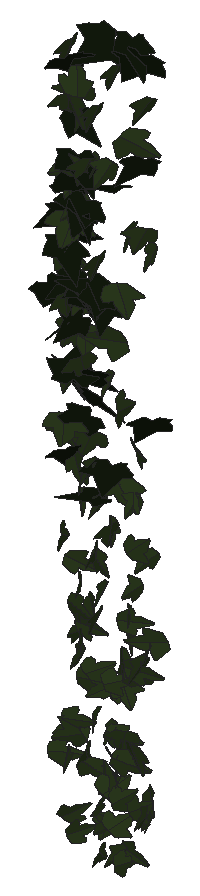
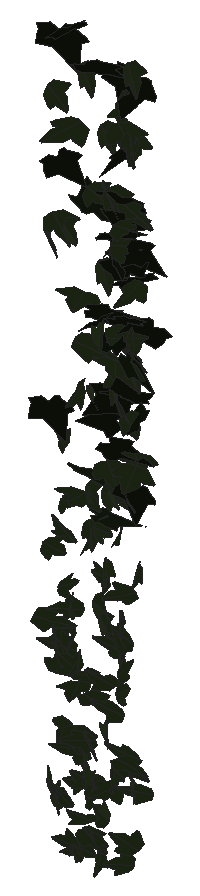
# SketchUp Ruby script. Lengths in inches.
U = 1.inch
M = Sketchup.active_model
def pt(a) = Geom::Point3d.new(a.map { |v| v * U })
def face(e, loops, mat)
  f = e.add_face(loops[0].map { |a| pt(a) })
  loops[1..].each { |l| e.add_face(l.map { |a| pt(a) }).erase! }
  f.material = f.back_material = mat if mat
  f
end
# faces: each face lists its corners as indices into pts; further lists are holes
def faces(e, pts, list, mat = nil) = list.each { |f| face(e, (f[0].is_a?(Array) ? f : [f]).map { |l| l.map { |i| pts[i] } }, mat) }
# xy, xz, yz: faces in a plane at the given z, y or x. An outline is a flat list of corners, or four numbers for a rectangle; further outlines are holes
def ring(l) = l.size == 4 ? [[l[0], l[1]], [l[2], l[1]], [l[2], l[3]], [l[0], l[3]]] : l.each_slice(2).to_a
def flat(e, list, mat, &to3) = list.each { |f| face(e, (f[0].is_a?(Array) ? f : [f]).map { |l| ring(l).map { |u, v| to3.(u, v) } }, mat) }
def xy(e, z, list, mat = nil) = flat(e, list, mat) { |x, y| [x, y, z] }
def xz(e, y, list, mat = nil) = flat(e, list, mat) { |x, z| [x, y, z] }
def yz(e, x, list, mat = nil) = flat(e, list, mat) { |y, z| [x, y, z] }
def lines(e, pts, list) = list.each { |a, b| e.add_line(pt(pts[a]), pt(pts[b])) }
# prism: a flat outline (further loops are holes) pulled along v
def prism(e, loops, v, mat = nil)
  f = face(e, loops, mat); d = Geom::Vector3d.new(v.map { |x| x * U })
  f.pushpull(f.normal.samedirection?(d) ? d.length : -d.length)
end
def box(e, o, s, mat = nil) = prism(e, [[o, [o[0] + s[0], o[1], o[2]], [o[0] + s[0], o[1] + s[1], o[2]], [o[0], o[1] + s[1], o[2]]]], [0, 0, s[2]], mat)
def at(x, y, z, deg = 0) = Geom::Transformation.translation(pt([x, y, z])) * Geom::Transformation.rotation(ORIGIN, Z_AXIS, deg.degrees)
def axes(o, x, y, z) = Geom::Transformation.new([*x, 0, *y, 0, *z, 0, *pt(o).to_a, 1])
def part(name) = M.definitions.add(name)
# library, detail: a bought-in or finely detailed component or shape, given as its bounding box
def library(name, o, s) = part(name).tap { |d| box(d.entities, o, s) }
def detail(e, o, s) = box(e.add_group.entities, o, s)
def put(e, d, t, mat = nil) = e.add_instance(d, t).tap { |i| i.material = mat if mat }
def group(e, t, mat = nil) = e.add_group.tap { |g| g.transformation = t; g.material = mat if mat }.entities
root = M.entities
M.materials.add("1026 AP 7946 SUNNY SIDE UP").color = [254, 231, 186]
M.materials.add("efeu1").color = [18, 25, 13]
M.materials.add("efeu2").color = [43, 57, 29]
c1 = part("ivyleaf_10")
p = [[0,0.5,-0.03],[-0.0625,2.02,-0.43],[-0.19,2.01,-0.46],[-0.54,1.05,-0.29],[-0.52,0.625,-0.18],[-0.83,0.76,-0.28],
  [-1.16,0.64,-0.33],[-1.15,0.33,-0.24],[-0.77,-0.39,0.02],[-0.3,-0.51,0.16],[0.04,-0.48,0.23],[-0.02,2.01,-0.4375],
  [-0.06,2.01,-0.43],[0.04,-0.49,0.23],[0.67,-0.49,0.14],[1.38,0.36,-0.2],[1.375,0.51,-0.24],[0.81,0.65,-0.19],
  [0.62,0.59,-0.15],[0.6,1.09,-0.28],[0.5,1.23,-0.31]]
faces(c1.entities,p,[[0,1,2,3,4,5,6,7,8,9,10],[11,12,0,13,14,15,16,17,18,19,20]],"efeu2")
c2 = part("ivyleaf_9")
p = [[1.54,2.16,1.25],[1.36,2.04,1.19],[-0.21,0.99,0.68],[-0.71,1.11,0.82],[-0.85,0.86,0.67],[-0.8,0.17,0.21],
  [-0.9,-0.01,0.1],[-0.67,-0.16,-0.02],[-0.08,-0.08,-0.05],[-0.03,-0.6,-0.4],[0.65,-0.88,-0.66],[0.83,-0.6,-0.49],
  [1.29,-0.42,-0.43],[1.8125,-0.07,-0.26],[1.21,0.44,0.15]]
faces(c2.entities,p,[[0,1,2,3,4,5,6,7,8,9,10,11,12,13,14]],"efeu1")
put(root,c1,axes([100.47,212.17,263.79],[-0.24039,0.02209,0.20935],[-0.32195,-0.07836,-0.13886],[0.08731,-0.22813,0.06438]),"1026 AP 7946 SUNNY SIDE UP")
put(root,c2,axes([99.98,211.93,261.11],[0.0239,-0.04755,-0.26687],[0.13435,0.23738,-0.04049],[0.40821,-0.07534,0.02895]),"1026 AP 7946 SUNNY SIDE UP")
put(root,c2,axes([100.4,212.09,262.84],[0.00155,0.07561,-0.24059],[-0.11917,-0.21559,-0.08063],[-0.38611,0.06685,0.02392]),"1026 AP 7946 SUNNY SIDE UP")
put(root,c2,axes([100.26,212.05,257.41],[0.11959,0.20678,-0.02726],[-0.00549,-0.02863,-0.23417],[-0.35421,0.07026,-0.00557]),"1026 AP 7946 SUNNY SIDE UP")
put(root,c2,axes([100.36,212.17,260.38],[-0.19771,0.17255,-0.11554],[0.07257,-0.10346,-0.2233],[-0.33987,-0.12247,0.01953]),"1026 AP 7946 SUNNY SIDE UP")
put(root,c1,axes([100.25,212.3,259.09],[-0.07215,-0.19809,0.09557],[0.0269,-0.09613,-0.21543],[0.36968,-0.03167,0.03433]),"1026 AP 7946 SUNNY SIDE UP")
put(root,c1,axes([100.21,212.19,257.9],[-0.32784,-0.10769,-0.06],[0.09966,0.00208,-0.24019],[0.16417,-0.2163,0.02598]),"1026 AP 7946 SUNNY SIDE UP")
put(root,c1,axes([100.26,211.95,255.57],[0.04261,-0.11798,-0.19372],[0.01525,0.18922,-0.12019],[0.34784,0.00616,0.029]),"1026 AP 7946 SUNNY SIDE UP")
put(root,c1,axes([100.26,212.12,265.35],[-0.149,-0.21531,-0.06932],[0.04877,0.05516,-0.24808],[0.37718,-0.09219,0.00469]),"1026 AP 7946 SUNNY SIDE UP")
put(root,c2,axes([100.03,212.26,259.12],[0.16229,-0.17368,0.11092],[0.07726,-0.09575,-0.2135],[0.33654,0.10573,-0.00448]),"1026 AP 7946 SUNNY SIDE UP")
put(root,c1,axes([100.07,212,250.61],[0.04726,-0.03496,-0.20865],[0.31184,0.05795,0.02037],[0.08369,-0.19618,0.04191]),"1026 AP 7946 SUNNY SIDE UP")
put(root,c1,axes([100.29,212,260.91],[-0.0584,-0.23989,-0.06459],[0.08038,0.05026,-0.25542],[0.41085,-0.04393,0.04079]),"1026 AP 7946 SUNNY SIDE UP")
put(root,c1,axes([100.34,212.1,260.19],[0.29929,-0.15384,-0.0563],[-0.03832,0.0507,-0.2486],[0.27222,0.17628,0.0269]),"1026 AP 7946 SUNNY SIDE UP")
put(root,c1,axes([100.56,212.04,251.13],[-0.15865,-0.02106,0.18555],[-0.25796,-0.07753,-0.1044],[0.12193,-0.19145,0.02055]),"1026 AP 7946 SUNNY SIDE UP")
put(root,c1,axes([100.27,212,258.12],[0.35327,0.11008,-0.0093],[0.00151,-0.02324,-0.25137],[-0.18764,0.20705,-0.01953]),"1026 AP 7946 SUNNY SIDE UP")
put(root,c1,axes([100.47,212.24,265.53],[-0.2725,-0.1754,0.07998],[-0.07203,-0.0654,-0.25513],[0.3171,-0.16559,0.01078]),"1026 AP 7946 SUNNY SIDE UP")
put(root,c1,axes([100.48,212.18,251.27],[0.22898,0.02611,-0.15658],[-0.22621,-0.05286,-0.15151],[-0.08799,0.20386,-0.01794]),"1026 AP 7946 SUNNY SIDE UP")
put(root,c1,axes([100.4,212.39,263.43],[-0.14982,-0.09397,0.20911],[0.02605,-0.22348,-0.09962],[0.3515,-0.02349,0.09651]),"1026 AP 7946 SUNNY SIDE UP")
put(root,c1,axes([100.46,211.84,250.5],[0.13131,-0.0727,0.19088],[-0.16696,0.15421,0.11228],[-0.26543,-0.13296,0.0238]),"1026 AP 7946 SUNNY SIDE UP")
put(root,c1,axes([100.65,212.21,260.78],[-0.07244,-0.03101,-0.23099],[-0.35299,-0.05878,0.05235],[-0.10871,0.21153,-0.01608]),"1026 AP 7946 SUNNY SIDE UP")
put(root,c2,axes([100.5625,212.23,261.22],[-0.33259,-0.07967,0.07775],[-0.09386,-0.0575,-0.22484],[0.15848,-0.20126,0.02999]),"1026 AP 7946 SUNNY SIDE UP")
put(root,c1,axes([100.58,212.04,265.14],[0.11068,-0.10389,-0.24427],[-0.18526,0.19894,-0.12835],[0.38082,0.12697,0.00855]),"1026 AP 7946 SUNNY SIDE UP")
put(root,c1,axes([100.32,211.96,261.91],[-0.07184,-0.17471,-0.19224],[0.19427,0.14977,-0.17567],[0.35059,-0.11879,0.05795]),"1026 AP 7946 SUNNY SIDE UP")
put(root,c1,axes([100.48,211.93,266.74],[-0.01419,-0.25609,-0.00995],[0.00654,0.00583,-0.2742],[0.43479,-0.00845,0.0038]),"1026 AP 7946 SUNNY SIDE UP")
put(root,c2,axes([100.29,212.04,263.29],[-0.0241,-0.02577,0.25431],[0.35854,0.11061,0.02787],[-0.19084,0.21107,0.02024]),"1026 AP 7946 SUNNY SIDE UP")
put(root,c1,axes([100.49,212.33,262.94],[-0.0328,-0.08521,0.26333],[0.01701,-0.25692,-0.08866],[0.42405,0.00371,0.02392]),"1026 AP 7946 SUNNY SIDE UP")
put(root,c1,axes([100.42,212.29,253.32],[-0.01623,0.05009,0.20745],[0.0955,-0.19176,0.0513],[0.31153,0.06139,-0.00492]),"1026 AP 7946 SUNNY SIDE UP")
put(root,c1,axes([100.43,212.01,262.68],[0.40722,0.09065,-0.04278],[-0.05012,-0.03574,-0.28189],[-0.14891,0.25992,-0.02211]),"1026 AP 7946 SUNNY SIDE UP")
put(root,c2,axes([100.34,211.98,262.12],[-0.06424,-0.24705,-0.07254],[0.05169,0.06426,-0.25666],[0.4,-0.04798,0.02152]),"1026 AP 7946 SUNNY SIDE UP")
put(root,c1,axes([100.53,212.17,254.51],[0.09787,-0.17064,-0.11209],[-0.00591,0.11184,-0.18391],[0.31734,0.05471,0.03114]),"1026 AP 7946 SUNNY SIDE UP")
put(root,c1,axes([100.4,211.98,249.29],[-0.0931,-0.13216,0.15943],[0.11063,0.13877,0.14991],[-0.30122,0.09182,0.00578]),"1026 AP 7946 SUNNY SIDE UP")
put(root,c2,axes([100.36,212.13,262.34],[0.38714,0.04627,0.03289],[-0.06485,0.03984,0.24472],[0.06766,-0.22656,0.04636]),"1026 AP 7946 SUNNY SIDE UP")
put(root,c2,axes([100.52,211.75,266.44],[0.22132,0.24374,0.02587],[0.03624,0.01235,-0.29543],[-0.4137,0.13148,-0.01204]),"1026 AP 7946 SUNNY SIDE UP")
put(root,c2,axes([100.75,212.17,258.3],[-0.02686,-0.00942,-0.22787],[-0.18564,-0.18267,0.01481],[-0.31015,0.11015,0.01087]),"1026 AP 7946 SUNNY SIDE UP")
put(root,c1,axes([100.33,212.23,257.1875],[0.19662,-0.05509,0.1929],[0.25585,-0.09406,-0.14077],[0.17035,0.20486,-0.01123]),"1026 AP 7946 SUNNY SIDE UP")
put(root,c2,axes([100.65,212.05,260.53],[-0.36307,0.03551,-0.07025],[0.10461,-0.03066,-0.23162],[-0.07261,-0.22175,0.01754]),"1026 AP 7946 SUNNY SIDE UP")
put(root,c1,axes([100.5,212.27,256.44],[-0.04039,0.17539,-0.09141],[0.00758,-0.08781,-0.19058],[-0.33277,-0.02329,0.00676]),"1026 AP 7946 SUNNY SIDE UP")
put(root,c1,axes([100.48,212.27,252.85],[0.03538,-0.04601,0.21155],[0.11769,-0.19155,-0.05372],[0.30969,0.07805,-0.00376]),"1026 AP 7946 SUNNY SIDE UP")
put(root,c2,axes([100.44,212.1,265.03],[0.12179,-0.15537,-0.19879],[-0.09068,0.17658,-0.1798],[0.39818,0.08774,0.01986]),"1026 AP 7946 SUNNY SIDE UP")
put(root,c1,axes([100.51,212.29,259.38],[0.23502,-0.16838,0.0621],[0.07114,-0.04347,-0.23393],[0.29509,0.14458,0.00693]),"1026 AP 7946 SUNNY SIDE UP")
put(root,c1,axes([100.49,212.04,248.88],[-0.02341,-0.05076,0.21508],[0.05491,0.20622,0.05535],[-0.3338,0.03748,-0.00598]),"1026 AP 7946 SUNNY SIDE UP")
put(root,c1,axes([100.33,212.11,251.39],[0.0679,-0.02737,-0.20279],[0.30645,-0.03279,0.04859],[-0.05993,-0.19869,0.0187]),"1026 AP 7946 SUNNY SIDE UP")
put(root,c1,axes([100.46,212.02,265.41],[-0.23187,0.12601,-0.18662],[0.1617,-0.15184,-0.19769],[-0.32989,-0.16299,0.03427]),"1026 AP 7946 SUNNY SIDE UP")
put(root,c2,axes([100.46,212.24,264],[-0.18607,-0.14586,-0.17054],[0.22742,0.09156,-0.18943],[0.28456,-0.16854,0.03988]),"1026 AP 7946 SUNNY SIDE UP")
put(root,c1,axes([100.43,212.07,255.02],[0.0934,0.06572,0.18877],[0.18654,0.13681,-0.08984],[-0.25763,0.12288,0.00339]),"1026 AP 7946 SUNNY SIDE UP")
put(root,c2,axes([100.64,212.18,262.625],[-0.20529,0.07403,-0.21494],[0.22221,-0.15821,-0.14837],[-0.2893,-0.17405,0.03857]),"1026 AP 7946 SUNNY SIDE UP")
put(root,c2,axes([100.64,211.875,259.27],[-0.33488,-0.01147,0.15683],[0.23427,0.0419,0.21813],[-0.05285,0.25845,-0.02684]),"1026 AP 7946 SUNNY SIDE UP")
put(root,c1,axes([100.71,212.2,263.97],[-0.10908,-0.23774,0.0525],[-0.01238,-0.05202,-0.26429],[0.41299,-0.06435,0.00594]),"1026 AP 7946 SUNNY SIDE UP")
put(root,c1,axes([100.76,212.27,257.83],[-0.29503,-0.13804,0.0738],[-0.06391,-0.06608,-0.23864],[0.23662,-0.18996,0.02756]),"1026 AP 7946 SUNNY SIDE UP")
put(root,c1,axes([100.4375,212.12,253.99],[-0.01408,-0.00289,-0.23559],[0.25744,-0.15985,-0.00546],[-0.25105,-0.16376,0.00761]),"1026 AP 7946 SUNNY SIDE UP")
put(root,c1,axes([100.67,211.89,265.78],[0.13771,0.24442,-0.09806],[0.03122,0.09367,0.27675],[0.44393,-0.08241,0.01096]),"1026 AP 7946 SUNNY SIDE UP")
put(root,c2,axes([100.68,212.17,263.09],[-0.24127,-0.20237,0.0063],[0.01145,-0.01514,-0.26452],[0.34364,-0.14158,0.01324]),"1026 AP 7946 SUNNY SIDE UP")
put(root,c2,axes([100.67,212.27,260.58],[0.23517,-0.16481,0.03448],[-0.01012,0.03965,0.22998],[-0.28561,-0.13711,0.02023]),"1026 AP 7946 SUNNY SIDE UP")
put(root,c2,axes([100.54,212.23,262.93],[0.04463,-0.23306,0.07772],[0.00252,-0.07592,-0.25205],[0.41594,0.02547,-0.00681]),"1026 AP 7946 SUNNY SIDE UP")
put(root,c1,axes([100.62,212.2,260.18],[0.36759,0.06433,0.0292],[0.04917,-0.00845,-0.24927],[-0.09874,0.23529,-0.01545]),"1026 AP 7946 SUNNY SIDE UP")
put(root,c1,axes([100.79,211.91,259.68],[-0.15743,-0.22993,-0.08635],[0.08127,0.06722,-0.25718],[0.37543,-0.11097,0.01946]),"1026 AP 7946 SUNNY SIDE UP")
put(root,c1,axes([100.68,212.02,253.39],[0.03429,-0.03152,0.1848],[0.18182,-0.13595,-0.0418],[0.23682,0.10894,0.00533]),"1026 AP 7946 SUNNY SIDE UP")
put(root,c1,axes([100.84,212.25,264.02],[0.19062,-0.22478,-0.01751],[-0.0345,0.00482,-0.26838],[0.38069,0.11299,-0.01555]),"1026 AP 7946 SUNNY SIDE UP")
put(root,c1,axes([100.83,211.98,250.86],[-0.00255,-0.16692,-0.14791],[0.00406,0.1426,-0.17113],[0.3452,-0.00291,0.00092]),"1026 AP 7946 SUNNY SIDE UP")
put(root,c1,axes([100.67,212.19,257.03],[0.09259,-0.15834,-0.12309],[0.11241,-0.09514,0.17575],[-0.3104,-0.08169,0.02693]),"1026 AP 7946 SUNNY SIDE UP")
put(root,c1,axes([100.83,212.24,257.21],[0.03266,-0.14537,0.187],[0.05189,-0.1794,-0.15225],[0.36299,0.03872,0.00494]),"1026 AP 7946 SUNNY SIDE UP")
put(root,c2,axes([101.08,212.17,256.6],[-0.34654,0.07741,-0.0097],[-0.09061,-0.159,-0.15225],[-0.09668,-0.12844,0.17744]),"1026 AP 7946 SUNNY SIDE UP")
put(root,c2,axes([101.15,212.22,261.21],[-0.14527,-0.13387,-0.19396],[-0.20911,-0.13399,0.16526],[-0.29584,0.16045,-0.02157]),"1026 AP 7946 SUNNY SIDE UP")
put(root,c1,axes([100.61,212.23,252.34],[0.04063,-0.02163,-0.21111],[0.31497,-0.04529,0.03069],[-0.07519,-0.2014,0.01452]),"1026 AP 7946 SUNNY SIDE UP")
put(root,c1,axes([100.71,212.24,254.1],[0.14483,-0.06109,0.20967],[0.25732,-0.12171,-0.11445],[0.21397,0.18771,-0.00429]),"1026 AP 7946 SUNNY SIDE UP")
put(root,c2,axes([100.74,212,259.3],[0.31039,0.10391,0.08075],[0.12335,0.02162,-0.22419],[-0.17807,0.19609,-0.01454]),"1026 AP 7946 SUNNY SIDE UP")
put(root,c1,axes([100.96,212.14,265.3],[-0.00566,-0.24071,0.05516],[0.00989,-0.05499,-0.24822],[0.38809,-0.00211,0.00713]),"1026 AP 7946 SUNNY SIDE UP")
put(root,c1,axes([100.68,212.06,253.65],[-0.04479,0.01446,0.22251],[0.3391,0.01986,0.02806],[-0.02807,0.21687,-0.01612]),"1026 AP 7946 SUNNY SIDE UP")
put(root,c1,axes([100.8,212.12,250.51],[-0.18042,-0.06463,-0.16258],[0.24131,0.0428,-0.13307],[0.1157,-0.19006,0.02402]),"1026 AP 7946 SUNNY SIDE UP")
put(root,c1,axes([100.96,212.34,256.41],[0.03485,-0.12368,0.17542],[0.05198,-0.16777,-0.13041],[0.32772,0.03976,0.00203]),"1026 AP 7946 SUNNY SIDE UP")
put(root,c1,axes([101.04,211.98,255.41],[0.01597,-0.16663,-0.15749],[-0.0061,0.15193,-0.17104],[0.35452,0.01012,0.00415]),"1026 AP 7946 SUNNY SIDE UP")
put(root,c2,axes([101.18,212.39,266.81],[-0.38858,-0.12684,0.08512],[-0.09578,-0.06297,-0.28517],[0.21858,-0.25308,0.02636]),"1026 AP 7946 SUNNY SIDE UP")
put(root,c1,axes([100.93,212.16,251.62],[-0.02103,-0.05833,-0.21353],[0.07486,-0.203,0.05459],[-0.32968,-0.04237,0.02602]),"1026 AP 7946 SUNNY SIDE UP")
put(root,c2,axes([100.76,212.11,258.83],[0.31358,-0.07471,0.09226],[0.12838,-0.04502,-0.21355],[0.1466,0.19923,-0.01035]),"1026 AP 7946 SUNNY SIDE UP")
put(root,c1,axes([101.125,212.34,263.97],[-0.11758,-0.16293,0.16557],[0.02477,-0.17325,-0.17341],[0.36003,-0.04129,0.066]),"1026 AP 7946 SUNNY SIDE UP")
put(root,c1,axes([101.04,212.25,260.58],[-0.01526,-0.12884,-0.20369],[0.01489,-0.19721,0.13125],[-0.36982,-0.00262,0.01369]),"1026 AP 7946 SUNNY SIDE UP")
put(root,c1,axes([101.16,211.96,262.07],[-0.01048,-0.26261,0.00476],[0.0037,-0.00617,-0.27065],[0.41302,-0.00661,0.00254]),"1026 AP 7946 SUNNY SIDE UP")
put(root,c1,axes([101.17,211.95,254.11],[0.06705,-0.22729,0.02985],[0.00144,-0.03061,-0.23837],[0.36055,0.04239,-0.0046]),"1026 AP 7946 SUNNY SIDE UP")
put(root,c2,axes([101.06,212.25,261.04],[-0.07893,-0.26405,0.05417],[-0.00761,-0.05412,-0.27716],[0.42375,-0.05016,0.00511]),"1026 AP 7946 SUNNY SIDE UP")
put(root,c1,axes([100.99,212.14,255.22],[-0.11117,0.03649,-0.20873],[0.1955,-0.16344,-0.0759],[-0.25841,-0.13935,0.03237]),"1026 AP 7946 SUNNY SIDE UP")
put(root,c1,axes([101.13,212.2,254.6],[0.05246,-0.14205,0.15137],[0.0728,-0.14059,-0.15085],[0.31394,0.05634,0.00969]),"1026 AP 7946 SUNNY SIDE UP")
put(root,c1,axes([101.14,211.93,249.66],[0.08173,-0.17897,0.11557],[-0.03654,0.11104,0.19249],[-0.33098,-0.05645,0.00729]),"1026 AP 7946 SUNNY SIDE UP")
put(root,c1,axes([101.32,212.16,252.43],[0.22782,0.03247,-0.15643],[-0.2216,-0.0603,-0.15198],[-0.1032,0.20117,-0.01899]),"1026 AP 7946 SUNNY SIDE UP")
put(root,c1,axes([101,211.97,252.74],[0.18413,0.01874,-0.17124],[0.24713,0.05751,0.12101],[0.09053,-0.19511,0.01797]),"1026 AP 7946 SUNNY SIDE UP")
put(root,c1,axes([101.39,212.17,249.3125],[-0.21401,-0.04306,0.15057],[-0.20539,-0.06855,-0.14627],[0.12406,-0.18777,0.01757]),"1026 AP 7946 SUNNY SIDE UP")
put(root,c1,axes([101.51,212.11,260.28],[0.12167,-0.01182,-0.27441],[-0.41672,0.02633,-0.08038],[0.04495,0.27606,-0.00246]),"1026 AP 7946 SUNNY SIDE UP")
put(root,c1,axes([101.24,211.92,248.75],[-0.01027,-0.13764,-0.15454],[0.02501,0.1485,-0.14095],[0.31823,-0.01611,0.00609]),"1026 AP 7946 SUNNY SIDE UP")
put(root,c1,axes([101.22,212.2,249.36],[0.29963,-0.07103,-0.00428],[-0.01418,-0.01348,-0.20895],[0.11095,0.19011,-0.01514]),"1026 AP 7946 SUNNY SIDE UP")
put(root,c1,axes([101.21,212.27,259.3],[0.19262,-0.17457,0.06891],[0.0379,-0.06574,-0.21938],[0.29207,0.12366,-0.01698]),"1026 AP 7946 SUNNY SIDE UP")
put(root,c2,axes([101.09,212.32,263.54],[-0.16853,-0.22391,0.02533],[0.37805,-0.10192,-0.03007],[0.05995,0.01324,0.26084]),"1026 AP 7946 SUNNY SIDE UP")
put(root,c1,axes([101.31,212.23,250.17],[-0.01215,0.0084,-0.20877],[-0.06932,-0.19807,-0.00789],[-0.31137,0.04377,0.0099]),"1026 AP 7946 SUNNY SIDE UP")
put(root,c1,axes([101.32,212.16,257.09],[0.03892,-0.19983,0.03775],[0.00696,-0.03752,-0.20765],[0.3197,0.02514,-0.00008]),"1026 AP 7946 SUNNY SIDE UP")
put(root,c1,axes([101.32,212.23,251.49],[0.17642,-0.17725,0.0029],[-0.01126,-0.00905,-0.21587],[0.27855,0.1119,-0.01056]),"1026 AP 7946 SUNNY SIDE UP")
put(root,c1,axes([101.26,212.28,256.04],[-0.033,0.17413,-0.13501],[0.02029,-0.13143,-0.18144],[-0.34302,-0.02452,0.00226]),"1026 AP 7946 SUNNY SIDE UP")
put(root,c1,axes([101.27,212.33,250.61],[-0.16766,0.06113,0.177],[0.19525,-0.12088,0.12324],[0.20929,0.16173,0.02682]),"1026 AP 7946 SUNNY SIDE UP")
put(root,c1,axes([101.48,211.91,250.375],[0.24303,-0.07393,0.14317],[-0.17979,0.08199,0.17589],[-0.17097,-0.19131,0.01856]),"1026 AP 7946 SUNNY SIDE UP")
put(root,c2,axes([101.34,212.15,257.38],[-0.30107,-0.16749,-0.08986],[0.29181,-0.1034,-0.17391],[0.12225,-0.16567,0.1938]),"1026 AP 7946 SUNNY SIDE UP")
put(root,c1,axes([101.47,211.96,256.13],[-0.06143,-0.22914,-0.02672],[0.01979,0.02282,-0.23917],[0.36184,-0.04015,0.00855]),"1026 AP 7946 SUNNY SIDE UP")
put(root,c1,axes([101.51,212.09,266.43],[-0.00327,-0.25152,0.02507],[0.00007,-0.02576,-0.25928],[0.39756,-0.00206,0.00025]),"1026 AP 7946 SUNNY SIDE UP")
put(root,c1,axes([101.6,211.89,250.47],[0.10369,-0.14529,-0.1596],[-0.11981,0.13431,-0.16327],[0.31072,0.10027,-0.00969]),"1026 AP 7946 SUNNY SIDE UP")
put(root,c1,axes([101.45,212.29,256.98],[-0.34916,-0.08936,-0.13161],[0.25605,-0.1108,-0.18726],[0.01336,-0.21179,0.1492]),"1026 AP 7946 SUNNY SIDE UP")
put(root,c1,axes([101.6875,211.96,251.23],[0.08712,-0.19475,-0.12677],[-0.05885,0.11612,-0.20788],[0.35648,0.06676,-0.00334]),"1026 AP 7946 SUNNY SIDE UP")
put(root,c1,axes([101.67,212.08,248.88],[-0.02012,-0.12237,0.1684],[-0.0118,-0.16409,-0.12758],[0.32174,-0.01367,0.00586]),"1026 AP 7946 SUNNY SIDE UP")
put(root,c1,axes([101.57,212.26,253.2],[-0.03728,0.19602,-0.12508],[0.01516,-0.12222,-0.20408],[-0.36316,-0.02522,0.00432]),"1026 AP 7946 SUNNY SIDE UP")
put(root,c1,axes([101.41,212.15,251.41],[-0.07569,-0.05101,-0.20562],[0.31011,0.04681,-0.06114],[0.09206,-0.19962,0.0369]),"1026 AP 7946 SUNNY SIDE UP")
put(root,c1,axes([101.72,212.12,251.48],[-0.24897,-0.13617,0.03029],[-0.01962,-0.03163,-0.21472],[0.21843,-0.15805,0.01523]),"1026 AP 7946 SUNNY SIDE UP")
put(root,c1,axes([101.51,211.85,250.29],[0.23172,0.05068,-0.17008],[0.19971,0.11579,0.15382],[0.18464,-0.18884,0.04707]),"1026 AP 7946 SUNNY SIDE UP")
put(root,c1,axes([101.53,212.15,261.41],[0.32279,0.12669,0.07464],[0.10952,0.02341,-0.24784],[-0.20102,0.21619,-0.01518]),"1026 AP 7946 SUNNY SIDE UP")
put(root,c1,axes([101.51,211.9,252.7],[0.11,0.001,-0.20078],[0.24614,0.12308,0.05925],[0.18258,-0.16652,0.04108]),"1026 AP 7946 SUNNY SIDE UP")
put(root,c1,axes([101.57,211.93,249.46],[0.2295,0.02298,-0.14895],[0.17748,0.11262,0.13636],[0.14692,-0.17194,0.06796]),"1026 AP 7946 SUNNY SIDE UP")
put(root,c1,axes([101.68,212.26,253.72],[-0.10047,0.17775,-0.07597],[0.02979,-0.07258,-0.19491],[-0.30174,-0.06635,0.00605]),"1026 AP 7946 SUNNY SIDE UP")
put(root,c1,axes([101.67,212.13,252.55],[0.18251,0.17702,0.03991],[0.04464,0.02647,-0.21772],[-0.28108,0.11915,-0.00866]),"1026 AP 7946 SUNNY SIDE UP")
put(root,c1,axes([101.75,212.15,252.93],[-0.05798,-0.16912,0.13107],[0.03404,0.12644,0.179],[-0.33195,0.04251,-0.00454]),"1026 AP 7946 SUNNY SIDE UP")
put(root,c1,axes([101.79,212.28,262.86],[0.07869,-0.20012,0.12508],[0.07134,-0.11469,-0.2127],[0.36202,0.0661,0.01473]),"1026 AP 7946 SUNNY SIDE UP")
put(root,c1,axes([101.83,212.32,256.73],[-0.08657,-0.10566,0.17077],[0.07246,-0.17484,-0.09971],[0.3013,0.01169,0.07304]),"1026 AP 7946 SUNNY SIDE UP")
put(root,c1,axes([101.84,211.79,259.01],[0.03339,-0.0751,-0.27636],[0.06988,0.26608,-0.07168],[0.43177,-0.03726,0.03297]),"1026 AP 7946 SUNNY SIDE UP")
put(root,c1,axes([101.87,212.3125,254.78],[-0.05571,-0.01829,0.21299],[0.05478,-0.20739,-0.01396],[0.32189,0.03213,0.03924]),"1026 AP 7946 SUNNY SIDE UP")
put(root,c2,axes([101.99,212.32,264.41],[0.00985,0.11519,-0.22163],[0.00406,-0.21588,-0.11991],[-0.3846,0.00067,-0.00694]),"1026 AP 7946 SUNNY SIDE UP")
put(root,c1,axes([101.79,211.85,248.73],[0.02061,-0.0044,-0.21517],[0.1617,0.18227,0.00377],[0.28589,-0.10278,0.01339]),"1026 AP 7946 SUNNY SIDE UP")
put(root,c1,axes([101.8,211.75,250.2],[0.06608,0.04454,-0.21364],[0.17191,0.17691,0.06293],[0.28625,-0.11653,0.01153]),"1026 AP 7946 SUNNY SIDE UP")
put(root,c1,axes([101.82,212.14,254.22],[0.00419,0.00105,0.2137],[0.18615,-0.17035,-0.00167],[0.26783,0.11838,-0.00218]),"1026 AP 7946 SUNNY SIDE UP")
put(root,c1,axes([101.71,211.97,250.99],[-0.04922,-0.03641,-0.22745],[0.35147,-0.00089,-0.03253],[0.00663,-0.22279,0.03597]),"1026 AP 7946 SUNNY SIDE UP")
put(root,c1,axes([101.75,212.12,248.91],[0.05238,0.0021,0.2066],[0.31533,-0.00092,-0.03432],[0.00088,0.20328,-0.0011]),"1026 AP 7946 SUNNY SIDE UP")
put(root,c1,axes([101.83,211.98,254.15],[-0.0193,0.01292,0.21732],[0.17934,0.17821,-0.00336],[-0.27963,0.1134,-0.01715]),"1026 AP 7946 SUNNY SIDE UP")
put(root,c1,axes([102.08,212.15,252.81],[-0.19544,-0.16721,-0.0414],[-0.0543,-0.02312,0.21404],[-0.26455,0.12827,-0.01334]),"1026 AP 7946 SUNNY SIDE UP")
put(root,c1,axes([102.16,212.17,262.92],[-0.19642,-0.19064,0.08066],[-0.03305,-0.08055,-0.23385],[0.32302,-0.12416,0.02512]),"1026 AP 7946 SUNNY SIDE UP")
put(root,c1,axes([101.89,211.98,265],[-0.17073,-0.14583,-0.23621],[0.31336,0.12385,-0.17829],[0.28885,-0.22055,0.0538]),"1026 AP 7946 SUNNY SIDE UP")
put(root,c2,axes([101.97,212.07,267.23],[-0.01343,-0.2527,-0.04873],[0.01084,0.04565,-0.26016],[0.4037,-0.00963,0.00536]),"1026 AP 7946 SUNNY SIDE UP")
put(root,c1,axes([101.93,212.16,249.84],[0.21768,-0.07452,-0.14065],[0.20019,-0.04972,0.16117],[-0.13948,-0.18766,0.0118]),"1026 AP 7946 SUNNY SIDE UP")
put(root,c1,axes([102.1875,212.25,265.82],[-0.0363,-0.22227,0.11735],[-0.02326,-0.11425,-0.23087],[0.39294,-0.0273,-0.00282]),"1026 AP 7946 SUNNY SIDE UP")
put(root,c2,axes([102.25,211.94,267.01],[0.21534,0.11012,-0.2155],[-0.21509,-0.16112,-0.18005],[-0.30422,0.19187,-0.02523]),"1026 AP 7946 SUNNY SIDE UP")
put(root,c1,axes([102.09,211.93,251.375],[-0.29758,0.1291,-0.06996],[0.07119,-0.05502,-0.23551],[-0.21861,-0.19365,0.01854]),"1026 AP 7946 SUNNY SIDE UP")
put(root,c1,axes([101.96,212.05,255.76],[0.25359,-0.07848,-0.12046],[0.17748,-0.03315,0.1838],[-0.13145,-0.19616,0.01577]),"1026 AP 7946 SUNNY SIDE UP")
put(root,c1,axes([101.97,212.17,257.92],[-0.12029,0.01694,0.20828],[0.26575,-0.11404,0.07509],[0.17622,0.18353,0.02893]),"1026 AP 7946 SUNNY SIDE UP")
put(root,c1,axes([102.22,212.34,255.6],[-0.08528,-0.11458,0.17799],[-0.00975,-0.17826,-0.12437],[0.32669,-0.03523,0.04275]),"1026 AP 7946 SUNNY SIDE UP")
put(root,c2,axes([102.31,212.2,258.71],[0.07993,0.19104,-0.14704],[-0.06117,-0.13846,-0.20446],[-0.37099,0.06399,0.00203]),"1026 AP 7946 SUNNY SIDE UP")
put(root,c1,axes([102.23,212.03,253.35],[0.00515,-0.17515,0.15833],[0.03192,-0.1539,-0.18086],[0.36604,0.01588,0.01354]),"1026 AP 7946 SUNNY SIDE UP")
put(root,c1,axes([102.22,212.125,249.85],[0.04179,-0.04305,0.20931],[0.10379,-0.19272,-0.05203],[0.31004,0.07032,-0.0108]),"1026 AP 7946 SUNNY SIDE UP")
put(root,c1,axes([102.5,212.2,253.82],[0.09969,-0.00325,-0.23782],[-0.34287,-0.07945,-0.06101],[-0.1192,0.22581,-0.0234]),"1026 AP 7946 SUNNY SIDE UP")
put(root,c1,axes([102.3125,212.25,262.54],[0.21082,-0.19484,0.00978],[-0.00361,-0.01443,-0.24352],[0.30679,0.13372,-0.00958]),"1026 AP 7946 SUNNY SIDE UP")
put(root,c1,axes([102.34,212.06,253.66],[0.11005,-0.18028,-0.06361],[-0.01574,0.06113,-0.19848],[0.29871,0.06964,0.01298]),"1026 AP 7946 SUNNY SIDE UP")
put(root,c1,axes([102.06,211.93,253.16],[-0.02458,-0.00019,0.23135],[0.32243,0.09179,0.01532],[-0.144,0.20555,-0.00518]),"1026 AP 7946 SUNNY SIDE UP")
put(root,c1,axes([102.375,212.05,249.89],[0.13137,-0.17968,-0.06891],[-0.05369,0.05672,-0.20369],[0.29609,0.09001,-0.00636]),"1026 AP 7946 SUNNY SIDE UP")
put(root,c1,axes([102.16,212.3,250.23],[0.14447,-0.0579,0.20472],[0.2481,-0.12168,-0.1122],[0.21141,0.18236,-0.00822]),"1026 AP 7946 SUNNY SIDE UP")
